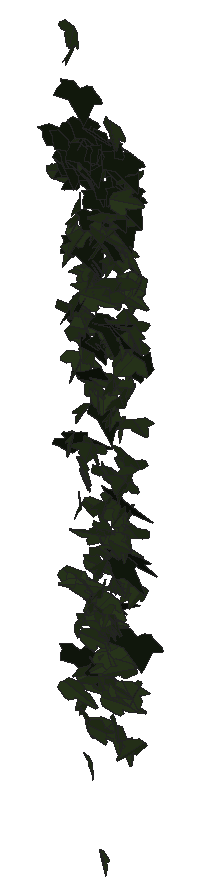
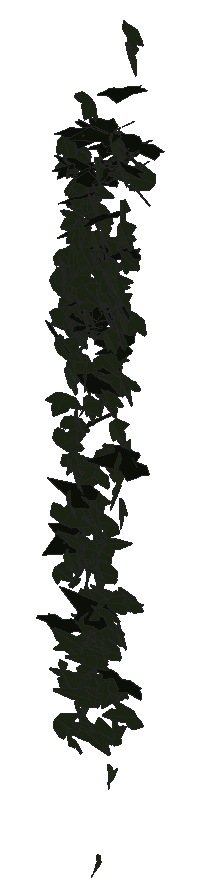
# SketchUp Ruby script. Lengths in millimetres.
U = 1.mm
M = Sketchup.active_model
def pt(a) = Geom::Point3d.new(a.map { |v| v * U })
def face(e, loops, mat)
  f = e.add_face(loops[0].map { |a| pt(a) })
  loops[1..].each { |l| e.add_face(l.map { |a| pt(a) }).erase! }
  f.material = f.back_material = mat if mat
  f
end
# faces: each face lists its corners as indices into pts; further lists are holes
def faces(e, pts, list, mat = nil) = list.each { |f| face(e, (f[0].is_a?(Array) ? f : [f]).map { |l| l.map { |i| pts[i] } }, mat) }
# xy, xz, yz: faces in a plane at the given z, y or x. An outline is a flat list of corners, or four numbers for a rectangle; further outlines are holes
def ring(l) = l.size == 4 ? [[l[0], l[1]], [l[2], l[1]], [l[2], l[3]], [l[0], l[3]]] : l.each_slice(2).to_a
def flat(e, list, mat, &to3) = list.each { |f| face(e, (f[0].is_a?(Array) ? f : [f]).map { |l| ring(l).map { |u, v| to3.(u, v) } }, mat) }
def xy(e, z, list, mat = nil) = flat(e, list, mat) { |x, y| [x, y, z] }
def xz(e, y, list, mat = nil) = flat(e, list, mat) { |x, z| [x, y, z] }
def yz(e, x, list, mat = nil) = flat(e, list, mat) { |y, z| [x, y, z] }
def lines(e, pts, list) = list.each { |a, b| e.add_line(pt(pts[a]), pt(pts[b])) }
# prism: a flat outline (further loops are holes) pulled along v
def prism(e, loops, v, mat = nil)
  f = face(e, loops, mat); d = Geom::Vector3d.new(v.map { |x| x * U })
  f.pushpull(f.normal.samedirection?(d) ? d.length : -d.length)
end
def box(e, o, s, mat = nil) = prism(e, [[o, [o[0] + s[0], o[1], o[2]], [o[0] + s[0], o[1] + s[1], o[2]], [o[0], o[1] + s[1], o[2]]]], [0, 0, s[2]], mat)
def at(x, y, z, deg = 0) = Geom::Transformation.translation(pt([x, y, z])) * Geom::Transformation.rotation(ORIGIN, Z_AXIS, deg.degrees)
def axes(o, x, y, z) = Geom::Transformation.new([*x, 0, *y, 0, *z, 0, *pt(o).to_a, 1])
def part(name) = M.definitions.add(name)
# library, detail: a bought-in or finely detailed component or shape, given as its bounding box
def library(name, o, s) = part(name).tap { |d| box(d.entities, o, s) }
def detail(e, o, s) = box(e.add_group.entities, o, s)
def put(e, d, t, mat = nil) = e.add_instance(d, t).tap { |i| i.material = mat if mat }
def group(e, t, mat = nil) = e.add_group.tap { |g| g.transformation = t; g.material = mat if mat }.entities
root = M.entities
M.materials.add("efeu1").color = [18, 25, 13]
M.materials.add("efeu2").color = [43, 57, 29]
c1 = part("ivyleaf_10")
p = [[0,12.8,-0.8],[-1.5,51.3,-10.9],[-4.9,51,-11.6],[-13.6,26.5,-7.3],[-13.2,15.9,-4.6],[-21.1,19.3,-7.2],
  [-29.5,16.3,-8.3],[-29.2,8.3,-6.2],[-19.7,-9.8,0.5],[-7.6,-13,4],[1,-12.2,5.8],[-0.4,51.1,-11.1],
  [-1.5,51.1,-10.9],[1,-12.4,5.9],[16.9,-12.4,3.5],[35.1,9.1,-5.1],[35,12.9,-6.1],[20.5,16.4,-4.9],
  [15.8,15,-3.8],[15.3,27.6,-7.1],[12.8,31.3,-7.8]]
faces(c1.entities,p,[[0,1,2,3,4,5,6,7,8,9,10],[11,12,0,13,14,15,16,17,18,19,20]],"efeu2")
c2 = part("ivyleaf_9")
p = [[39.1,54.8,31.7],[34.5,51.8,30.2],[-5.3,25.2,17.3],[-17.9,28.3,20.9],[-21.6,21.7,17],[-20.2,4.3,5.3],
  [-22.9,-0.3,2.5],[-17.1,-4,-0.6],[-2,-2.1,-1.2],[-0.7,-15.4,-10.1],[16.6,-22.3,-16.7],[21.1,-15.1,-12.5],
  [32.7,-10.7,-11],[46.1,-1.8,-6.6],[30.8,11.2,3.8]]
faces(c2.entities,p,[[0,1,2,3,4,5,6,7,8,9,10,11,12,13,14]],"efeu1")
put(root,c1,axes([1443.2,1009,891.5],[0.4432,-0.71141,0.02055],[0.0122,-0.01952,-0.74856],[1.35447,0.23296,0.00002]))
put(root,c1,axes([1420.9,977.9,1291.8],[0.03259,-0.22317,0.76558],[0.8664,0.63146,0.17389],[-1.2461,0.43321,0.14093]))
put(root,c2,axes([1421.4,989.4,1371.5],[-0.26237,-0.34361,-0.6958],[0.87628,0.53265,-0.35426],[1.18887,-0.46843,0.10756]))
put(root,c1,axes([1438.2,1034.8,194.6],[-0.19605,0.09852,0.6633],[0.4225,-0.62823,0.12779],[1.20428,0.23644,0.06315]))
put(root,c1,axes([1456.8,1015.2,448],[-0.06629,0.05289,0.64535],[-0.52427,-0.5861,0.03317],[1.11528,-0.27237,0.05395]))
put(root,c1,axes([1443.9,998.9,1135.7],[-0.06854,-0.55699,0.49682],[0.19163,-0.49647,-0.54931],[1.4075,0.04047,0.09898]))
put(root,c1,axes([1446.1,1007.6,1196.4],[0.07001,-0.74511,0.13637],[0.06701,-0.1347,-0.74549],[1.44009,0.04249,0.02806]))
put(root,c1,axes([1447.3,987,1547.4],[0.3478,-0.78477,-0.11098],[0.00279,0.11422,-0.80531],[1.50842,0.18073,0.02708]))
put(root,c2,axes([1467.9,980.6,1289.9],[-0.52167,0.59282,0.51746],[-0.42773,0.46615,-0.65309],[-1.43524,-0.3544,0.00655]))
put(root,c1,axes([1439,996.8,751.6],[0.58658,-0.50599,0.35522],[0.38482,-0.29258,-0.5922],[1.1119,0.36819,0.01756]))
put(root,c1,axes([1439.2,1019.2,902],[1.25724,0.17652,0.0558],[0.09848,0.02248,-0.68372],[-0.33829,0.66257,0.00833]))
put(root,c2,axes([1437.4,1001.9,1313.9],[-0.16929,-0.74088,0.20839],[-0.03156,-0.20788,-0.74616],[1.46443,-0.09013,0.00801]))
put(root,c1,axes([1422.4,1008.9,459.4],[0.55455,0.00595,0.60829],[1.15474,0.0458,-0.29108],[-0.0835,0.67292,0.01443]))
put(root,c2,axes([1425.5,1003,738.6],[0.25682,0.26931,-0.70933],[0.51907,0.65509,0.3006],[1.34751,-0.30367,0.0194]))
put(root,c1,axes([1442,991.5,1015.8],[-1.35528,0.1639,-0.25147],[0.45635,-0.07885,-0.7304],[-0.34365,-0.75107,0.02181]))
put(root,c1,axes([1452.2,1021,805.4],[-0.01871,-0.68823,0.14291],[-0.01415,-0.14281,-0.68828],[1.33771,-0.01114,-0.00528]))
put(root,c2,axes([1433.3,990.7,1314.8],[0.51571,-0.66444,-0.29611],[-0.05376,0.30614,-0.71279],[1.38342,0.25959,0.08268]))
put(root,c1,axes([1453.5,1005.5,982.2],[0.59287,-0.61086,-0.26841],[-0.11592,0.26895,-0.68278],[1.26457,0.31104,0.06325]))
put(root,c1,axes([1449.3,983.3,1585],[1.08412,-0.56149,-0.18704],[0.0272,0.27258,-0.77474],[1.12603,0.534,0.1988]))
put(root,c1,axes([1424,1011.9,231.1],[0.68955,0.00679,0.65215],[1.2245,0.11836,-0.35868],[-0.20312,0.73658,0.05162]))
put(root,c1,axes([1449.5,1001.3,1007.7],[0.76255,-0.54006,0.30653],[-0.24307,0.28533,0.66965],[-1.1566,-0.41603,0.06136]))
put(root,c2,axes([1434.8,990.2,1359.9],[0.2371,-0.77171,-0.14079],[0.19691,0.15748,-0.7716],[1.47991,0.10269,0.12522]))
put(root,c2,axes([1433,1013.4,969.4],[1.01094,-0.5476,0.02157],[0.02226,-0.01871,-0.76288],[1.04276,0.53129,-0.00463]))
put(root,c1,axes([1453.9,1002.9,1322.6],[0.39172,-0.74294,0.04333],[0.10233,-0.03,-0.76968],[1.41266,0.20819,0.04374]))
put(root,c2,axes([1468.2,1003.6,1319.6],[-1.41199,-0.19795,0.05758],[-0.10372,-0.01909,-0.76784],[0.3784,-0.74389,0.00438]))
put(root,c1,axes([1456,1010.5,674],[-0.48892,0.64643,0.18666],[-0.16992,0.16529,-0.69528],[-1.26923,-0.27114,0.02118]))
put(root,c2,axes([1441.8,1020,303.6],[-0.746,-0.20725,-0.62022],[1.0269,0.30604,-0.44326],[0.70316,-0.66683,-0.01067]))
put(root,c1,axes([1455.5,995.9,1234.3],[0.24112,-0.69615,-0.24596],[0.16234,0.26168,-0.69672],[1.39577,0.08983,0.12353]))
put(root,c1,axes([1460.2,1025.4,1102.2],[0.40735,-0.68514,0.11083],[0.02592,-0.11181,-0.71751],[1.32066,0.21352,-0.0201]))
put(root,c1,axes([1449.2,1004.2,369.6],[0.15642,-0.45535,-0.49981],[0.2751,-0.48002,0.46109],[-1.25707,-0.16171,0.03871]))
put(root,c1,axes([1456.4,992.5,1040.5],[0.26204,-0.65321,0.33663],[0.28255,-0.3107,-0.66361],[1.36972,0.18905,0.07249]))
put(root,c1,axes([1458.9,995.4,1166.7],[0.00847,-0.57781,0.48339],[0.20024,-0.47819,-0.57256],[1.41973,0.07089,0.07787]))
put(root,c1,axes([1463.4,1004.9,1371.8],[-0.03206,-0.77554,0.00348],[-0.00159,-0.00347,-0.77572],[1.47602,-0.01685,-0.00076]))
put(root,c2,axes([1466.8,989.6,1042.7],[-0.93135,0.42308,-0.43345],[0.63516,-0.27669,-0.64685],[-0.962,-0.59228,-0.00744]))
put(root,c1,axes([1464.8,1015.5,1090.7],[-0.5575,-0.65264,0.18639],[0.01094,-0.20539,-0.71012],[1.29172,-0.27994,0.08646]))
put(root,c1,axes([1469.6,1025.7,936.8],[-0.83095,-0.41397,0.34569],[-0.15031,-0.3909,-0.56786],[1.01538,-0.39665,0.19884]))
put(root,c1,axes([1466.1,985.2,628.7],[0.25675,-0.53892,-0.51614],[-0.03387,0.52204,-0.54972],[1.41979,0.10991,0.08022]))
put(root,c1,axes([1453,996.3,1160.3],[0.54011,0.33168,-0.70111],[0.64999,0.61686,0.43006],[1.32533,-0.4377,0.07481]))
put(root,c1,axes([1467.3,1019.1,980.4],[0.01607,-0.68794,0.11701],[-0.0117,-0.11709,-0.68796],[1.32805,0.00729,-0.00748]))
put(root,c1,axes([1462.8,1018.1,279.2],[-0.57389,-0.58911,-0.31887],[0.34056,0.26614,-0.66091],[1.22857,-0.34896,0.03425]))
put(root,c2,axes([1447.4,992.8,1331.5],[0.59078,-0.69709,-0.19095],[0.0923,0.22743,-0.75145],[1.37248,0.28476,0.13273]))
put(root,c2,axes([1450.1,986.5,1336.5],[0.43371,-0.68741,-0.30167],[0.05207,0.32266,-0.71457],[1.42777,0.19705,0.1177]))
put(root,c1,axes([1469.5,999.9,1006.1],[0.86428,-0.56948,-0.07185],[-0.07097,0.06215,-0.72831],[1.09011,0.45555,0.00954]))
put(root,c1,axes([1475.5,1008.4,737.3],[-0.99607,-0.46039,0.09507],[-0.1241,-0.06981,-0.69698],[0.88606,-0.52733,0.00926]))
put(root,c1,axes([1462.7,1013.8,1085.4],[-0.32445,0.66531,-0.22893],[0.11537,-0.22079,-0.68679],[-1.3341,-0.1809,-0.00372]))
put(root,c1,axes([1487.9,1013.6,558.6],[-0.26023,0.03474,-0.62065],[-1.07167,-0.27614,0.1086],[-0.5012,0.57241,0.09006]))
put(root,c2,axes([1461.7,992.9,1465.5],[-0.48078,-0.74161,-0.16443],[0.08133,0.15913,-0.78339],[1.44343,-0.25599,-0.01063]))
put(root,c1,axes([1458.7,1001,702.2],[-0.48312,0.46249,-0.49972],[0.4288,-0.44622,-0.52742],[-1.22288,-0.33918,0.01248]))
put(root,c1,axes([1460.7,1011.9,743.4],[-0.78915,0.50002,-0.3271],[0.4121,-0.24533,-0.64952],[-1.05988,-0.46769,-0.009]))
put(root,c1,axes([1472.6,1018.6,860.6],[1.10535,-0.27628,-0.20982],[-0.22778,0.22448,-0.62686],[0.61972,0.57528,0.14384]))
put(root,c2,axes([1486,993,1356.5],[-1.44087,0.20191,-0.12469],[0.21102,-0.06762,-0.7827],[-0.39932,-0.76429,0.03631]))
put(root,c1,axes([1471.9,1004.8,1114.1],[-0.85937,0.56141,0.074],[-0.0993,0.05299,-0.72043],[-1.07314,-0.45448,0.0074]))
put(root,c1,axes([1475.5,1020.7,1071.7],[-0.14093,-0.71007,0.10685],[-0.01513,-0.1066,-0.71392],[1.36654,-0.07441,0.00311]))
put(root,c1,axes([1443.7,1005.6,450.6],[0.39134,-0.11436,-0.72012],[1.37291,-0.07706,0.21822],[-0.20209,-0.74493,0.08798]))
put(root,c1,axes([1462.2,1007.3,180.6],[-0.59651,0.28867,0.50802],[0.71319,-0.34302,0.4261],[0.85325,0.48853,-0.001]))
put(root,c1,axes([1459.8,983,987.9],[-0.34796,-0.34077,-0.73583],[0.89725,0.56905,-0.38067],[1.25569,-0.50105,0.06811]))
put(root,c1,axes([1477.3,999.5,934.4],[0.79729,-0.48326,-0.26997],[-0.177,0.27231,-0.63176],[1.03856,0.4174,0.09958]))
put(root,c1,axes([1469.5,992,1330.6],[0.10412,0.76286,-0.02279],[-0.00187,-0.02278,-0.76482],[-1.45253,0.05471,-0.00065]))
put(root,c2,axes([1458.1,1003,1393.3],[0.49907,-0.67127,-0.29909],[-0.00908,0.316,-0.71341],[1.39861,0.24158,0.10209]))
put(root,c2,axes([1463.1,1003.5,1149.9],[-0.50102,-0.56288,-0.47031],[0.43311,0.41236,-0.62089],[1.32712,-0.34707,0.02507]))
put(root,c1,axes([1475.3,1025.1,1038.3],[0.68222,-0.60648,0.06114],[0.04696,-0.05643,-0.70446],[1.15916,0.35923,-0.00744]))
put(root,c1,axes([1482.4,1003.4,1068.7],[-0.67489,-0.56352,0.25401],[-0.11591,-0.25957,-0.66086],[1.17069,-0.35056,0.081]))
put(root,c1,axes([1476.9,1006,1117.6],[-0.9642,0.51359,0.07012],[-0.08621,0.05381,-0.72139],[-0.98276,-0.50861,-0.00551]))
put(root,c2,axes([1491.3,990.5,962.7],[0.68822,0.02148,-0.6927],[-1.31893,0.00382,-0.36165],[-0.01246,0.7814,0.02081]))
put(root,c1,axes([1483.7,1006,1106.7],[-0.57669,-0.61327,0.24037],[0.03656,-0.2727,-0.67153],[1.25309,-0.27428,0.13021]))
put(root,c1,axes([1488.3,1018.1,422.3],[1.13171,-0.21924,-0.29688],[-0.5257,0.10899,-0.63374],[0.46583,0.65563,0.00608]))
put(root,c1,axes([1481.8,1015.4,569.2],[-0.55508,0.60031,0.10335],[-0.11172,0.08635,-0.66724],[-1.15392,-0.29713,0.01489]))
put(root,c1,axes([1487.9,1014.6,1107.6],[-0.31374,-0.63964,0.30856],[-0.07828,-0.30763,-0.65969],[1.34933,-0.16657,0.03347]))
put(root,c1,axes([1485.5,1012,1184],[0.37967,-0.73235,-0.03365],[-0.01388,0.03289,-0.75903],[1.3952,0.19962,0.00161]))
put(root,c1,axes([1471.5,1011.4,87.9],[-0.37319,0.0677,0.65477],[0.77471,-0.52445,0.17612],[0.98456,0.43833,0.10961]))
put(root,c1,axes([1461.5,1024.7,608.7],[-0.39439,0.09072,-0.63142],[1.07466,-0.2828,-0.22595],[-0.56485,-0.60139,0.011]))
put(root,c1,axes([1480.3,1008.4,1095.9],[0.37984,-0.57233,0.42674],[0.30425,-0.39602,-0.6059],[1.32421,0.25516,0.0168]))
put(root,c1,axes([1464.8,1012.2,254.8],[0.75976,0.02486,-0.58698],[1.00609,0.29446,0.37199],[0.4879,-0.64591,0.14699]))
put(root,c1,axes([1492.8,1000.3,834],[0.12538,0.27428,-0.67419],[-0.13268,0.67621,0.26829],[1.37888,0.04013,0.08712]))
put(root,c1,axes([1463.5,1021.7,276.7],[-0.29689,0.01189,0.72121],[1.34588,-0.14288,0.15531],[0.27052,0.72392,0.01881]))
put(root,c2,axes([1478.4,1012.4,871],[1.40141,0.00783,0.21599],[-0.41119,0.00592,0.73634],[0.01113,-0.76735,0.00788]))
put(root,c1,axes([1485,1005.2,427.6],[-0.18719,-0.24476,-0.67812],[0.44494,0.63659,-0.26367],[1.29794,-0.25352,-0.00741]))
put(root,c1,axes([1465,1011.4,347.2],[0.14727,0.00514,0.66847],[1.23433,0.16251,-0.07633],[-0.30835,0.65301,0.01374]))
put(root,c1,axes([1475.1,1010.3,390.4],[-1.05334,-0.08744,-0.51833],[0.97325,0.08463,-0.56031],[0.23153,-0.75353,-0.00279]))
put(root,c2,axes([1481.7,990.8,1348.4],[-0.33793,-0.71373,-0.27923],[0.11589,0.27258,-0.73546],[1.45401,-0.18761,-0.00628]))
put(root,c1,axes([1493.7,1011.5,269.6],[-1.06274,-0.41819,-0.1508],[0.23417,0.08727,-0.69762],[0.81301,-0.57178,0.00381]))
put(root,c1,axes([1497.7,997.5,1158.1],[0.25738,-0.7155,-0.24789],[-0.06821,0.24548,-0.72811],[1.43954,0.13956,0.00982]))
put(root,c1,axes([1501.8,1024.1,172.5],[1.15359,-0.02355,-0.29756],[-0.56599,0.01021,-0.60659],[0.04881,0.67515,-0.0012]))
put(root,c1,axes([1491.8,1023.6,842],[0.54627,0.59829,-0.1598],[-0.11876,-0.14729,-0.66353],[-1.17257,0.29364,-0.00724]))
put(root,c1,axes([1498.5,1016.7,1166.3],[0.12014,-0.75009,-0.02448],[0.00406,0.02474,-0.75273],[1.42832,0.06302,0.0042]))
put(root,c2,axes([1481.7,1004.6,1295.5],[0.22715,-0.70852,0.26439],[0.03081,-0.26521,-0.71802],[1.43895,0.11752,-0.02636]))
put(root,c2,axes([1481.7,1005.3,1213.4],[0.23488,-0.63823,-0.40495],[0.06589,0.41465,-0.64298],[1.43704,0.0853,0.09567]))
put(root,c2,axes([1475.9,1004.7,1382],[1.38059,-0.27976,-0.0358],[0.12212,0.25992,-0.73081],[0.52271,0.67819,0.26532]))
put(root,c1,axes([1518.2,1007.2,582.3],[-0.61481,0.10404,0.5461],[-0.98137,0.17997,-0.33931],[-0.3954,-0.60844,-0.00699]))
put(root,c1,axes([1473.8,1011.4,499.3],[0.02011,-0.04651,0.69636],[1.2907,0.16514,0.00074],[-0.31366,0.67658,0.04769]))
put(root,c1,axes([1508.2,1026.6,1063.5],[-0.70213,-0.51319,0.36236],[-0.17373,-0.37197,-0.61974],[1.18296,-0.35923,0.12406]))
put(root,c1,axes([1518.1,1007.9,361.1],[0.36364,-0.15762,-0.59616],[-0.85167,0.39397,-0.24758],[0.80746,0.48652,0.00734]))
put(root,c1,axes([1494.5,1001.7,491.6],[0.29916,-0.64001,-0.20308],[0.12189,-0.19332,0.65885],[-1.27208,-0.16904,0.01537]))
put(root,c2,axes([1490.4,1027.5,805.1],[-0.02816,-0.75112,0.18296],[0.02991,-0.18325,-0.75103],[1.47102,-0.01065,0.01877]))
put(root,c1,axes([1503.9,1005.3,1306.2],[0.23302,-0.73575,-0.17778],[0.0798,0.18641,-0.74258],[1.43837,0.10885,0.07]))
put(root,c1,axes([1506.1,1007.5,635.2],[-0.21553,-0.62591,-0.07851],[0.02056,0.07783,-0.63607],[1.2004,-0.11372,-0.0032]))
put(root,c1,axes([1497.3,1013.1,-87.4],[-0.1945,0.53332,-0.33609],[0.1251,-0.32961,-0.54301],[-1.19321,-0.12149,-0.00215]))
put(root,c1,axes([1508.6,1030.5,402.6],[-0.18708,-0.54603,0.41116],[-0.06292,-0.4111,-0.55386],[1.29936,-0.09852,0.03238]))
put(root,c1,axes([1486.5,988.4,1054.3],[0.30282,0.18928,0.74365],[0.69884,0.64809,-0.24353],[-1.28238,0.39788,0.0429]))
put(root,c1,axes([1483.9,1028,376.1],[-0.15756,0.07986,0.75173],[1.22412,-0.38991,0.11226],[0.75598,0.64801,-0.0251]))
put(root,c1,axes([1514.8,1021.8,310.1],[0.43215,0.3104,-0.62414],[-0.75259,-0.48321,-0.38418],[-1.09252,0.45564,0.01776]))
put(root,c1,axes([1483,1006.2,409.1],[-0.38011,-0.04855,0.73188],[1.32196,-0.25623,0.17255],[0.44852,0.71406,0.11168]))
put(root,c1,axes([1534,1009.7,882],[-0.02132,0.05609,-0.73815],[-1.39931,0.08515,0.01763],[0.16411,0.73331,0.05442]))
put(root,c1,axes([1499.2,1015.8,694.1],[-1.08527,0.08825,-0.28166],[0.51692,-0.08298,-0.57587],[-0.21991,-0.63057,0.03637]))
put(root,c1,axes([1512.9,999.6,513.5],[0.42357,-0.29941,0.51724],[-0.50566,0.44483,0.37182],[-1.01887,-0.34524,0.0305]))
put(root,c1,axes([1515.5,1020.5,631.1],[0.89421,-0.55043,-0.28111],[-0.35372,0.21094,-0.72368],[1.12184,0.50525,-0.00411]))
put(root,c1,axes([1513.4,1008.1,443.3],[1.14149,-0.08531,-0.20905],[-0.39464,0.02668,-0.60581],[0.17005,0.6346,-0.00263]))
put(root,c2,axes([1482.3,1019.8,415.5],[1.17273,0.35231,-0.28515],[0.45287,0.15814,0.70957],[0.73419,-0.6603,0.0178]))
put(root,c1,axes([1499,1008.4,537.1],[-0.85517,-0.1857,-0.41301],[0.71657,0.17006,-0.48609],[0.47884,-0.58614,-0.01018]))
put(root,c1,axes([1483.3,1008.4,388],[0.22875,-0.0061,-0.71282],[1.35553,0.03094,0.11983],[0.05614,-0.72222,0.01115]))
put(root,c2,axes([1516.6,1002,1373.3],[-1.34912,-0.15793,-0.29073],[0.56802,-0.00854,-0.72306],[0.27178,-0.76612,0.068]))
put(root,c1,axes([1511.5,1009.9,702.3],[-0.89861,0.42684,-0.06049],[0.07845,-0.0446,-0.63647],[-0.81672,-0.47392,0.00542]))
put(root,c2,axes([1530.3,1006.1,965.4],[-1.03263,-0.55871,0.11639],[0.17401,0.07342,0.77868],[-1.07213,0.55004,0.01428]))
put(root,c1,axes([1517.9,984.6,475.9],[-0.00354,-0.64236,-0.35691],[-0.0121,0.35691,-0.64233],[1.39852,0.00146,-0.00646]))
put(root,c1,axes([1518.3,1024.2,1128.3],[-0.18922,-0.68694,0.23503],[0.01772,-0.23841,-0.69288],[1.38167,-0.09102,0.04107]))
put(root,c1,axes([1518.9,994.5,524.8],[-0.11144,-0.77801,0.02963],[-0.00537,-0.0295,-0.78021],[1.48177,-0.05862,-0.0006]))
put(root,c1,axes([1487.3,1004.6,169.7],[0.00993,-0.07878,0.72989],[1.37415,0.13257,0.00915],[-0.25272,0.71777,0.07842]))
put(root,c1,axes([1509.9,1022.6,362.9],[-0.35789,0.38277,0.56609],[0.49151,-0.50379,0.42643],[1.20412,0.31941,-0.00581]))
put(root,c1,axes([1524.7,1002.4,1134.1],[0.3882,-0.51904,-0.48633],[-0.37634,0.44461,-0.55745],[1.30035,0.28363,-0.01615]))
put(root,c1,axes([1519.1,1008.7,1065.5],[-1.04563,-0.48068,-0.18892],[0.30424,0.10402,-0.72954],[0.93469,-0.57159,0.02611]))
put(root,c1,axes([1510.8,1002.9,390.1],[0.0365,0.05739,-0.63411],[0.60377,0.54919,0.0593],[1.05065,-0.31759,-0.01205]))
put(root,c1,axes([1528.1,999.8,479.2],[0.06242,-0.04201,0.63628],[-0.61092,0.54943,0.05282],[-1.04863,-0.32259,0.0071]))
put(root,c1,axes([1523.8,1009.5,823.7],[0.14199,-0.70159,0.00059],[-0.00104,-0.00065,-0.70554],[1.33526,0.07461,-0.00061]))
put(root,c1,axes([1525,985.5,1234.6],[0.31488,-0.61795,-0.45472],[-0.05748,0.45957,-0.63552],[1.45905,0.15146,0.07309]))
put(root,c1,axes([1501.5,1009.4,320.1],[-0.30363,-0.07535,-0.64788],[1.15621,0.2256,-0.17583],[0.45183,-0.62794,0.01457]))
put(root,c1,axes([1513,1008.1,323.4],[1.05123,0.28289,0.14096],[0.22932,0.07392,-0.62049],[-0.55611,0.56524,0.0106]))
put(root,c1,axes([1527.3,1000.3,986.9],[0.10977,-0.70058,-0.01657],[-0.01091,0.01616,-0.70294],[1.33367,0.05779,-0.00439]))
put(root,c1,axes([1517.7,990.6,1010.7],[0.92019,0.62664,0.04036],[0.04596,0.03235,-0.79148],[-1.1942,0.4841,0.00064]))
put(root,c1,axes([1526.5,1003.6,889.4],[0.06075,-0.68244,-0.38392],[0.15276,0.38507,-0.67781],[1.4824,-0.01171,0.08558]))
put(root,c1,axes([1526.8,1006.1,528.1],[0.02762,-0.12903,-0.69764],[0.14345,0.69412,-0.12681],[1.34262,-0.0715,0.0279]))
put(root,c1,axes([1522.8,1012.4,827.2],[-0.00911,0.48929,-0.55508],[-0.0284,-0.55505,-0.48912],[-1.40798,0.00803,0.01346]))
put(root,c1,axes([1528.9,992.9,1225.5],[0.65928,-0.69048,0.02761],[0.00542,-0.02945,-0.77243],[1.31517,0.34625,-0.01066]))
put(root,c1,axes([1531.1,1001.9,994.7],[0.68897,-0.59674,-0.17286],[-0.0847,0.17464,-0.69609],[1.17936,0.36115,0.05099]))
put(root,c2,axes([1508.4,995.4,991.8],[1.24413,0.41711,-0.05239],[0.08219,0.02971,0.77544],[0.79585,-0.65513,0.00182]))
put(root,c1,axes([1533.6,1018.9,1161.9],[-0.59508,-0.66254,-0.06306],[0.14295,0.0341,-0.73068],[1.25855,-0.31714,0.05317]))
put(root,c2,axes([1520.8,1001,1354.6],[-0.1036,-0.73111,-0.26218],[0.08047,0.25965,-0.73282],[1.47603,-0.06547,0.02155]))
put(root,c1,axes([1533.6,999.2,428.7],[0.40806,0.45945,-0.40181],[-0.30649,-0.36821,-0.50696],[-1.12049,0.26804,-0.00766]))
put(root,c2,axes([1519.5,997.1,1291.2],[0.29175,-0.69187,-0.32191],[-0.04731,0.32364,-0.70743],[1.45155,0.14961,0.04164]))
put(root,c2,axes([1520.1,990.6,1270.7],[-0.36739,-0.58333,-0.50813],[0.42136,0.46015,-0.61236],[1.41075,-0.28935,0.05057]))
put(root,c1,axes([1534.3,994.4,1415.2],[-1.10625,0.51723,-0.15152],[-0.01491,-0.23093,-0.75826],[-1.02565,-0.55452,0.17445]))
put(root,c1,axes([1509.3,988,1198.6],[-0.45728,0.08563,-0.74359],[1.36504,-0.19703,-0.25444],[-0.40744,-0.7562,-0.01791]))
put(root,c1,axes([1556.6,989.8,1141.6],[0.61275,-0.11346,0.72174],[-1.27889,0.2636,0.34119],[-0.54579,-0.74504,0.01081]))
put(root,c1,axes([1527.6,1030.5,796.3],[0.60292,-0.43259,0.41337],[0.47852,-0.32819,-0.53613],[1.03333,0.40438,0.00709]))
put(root,c1,axes([1514.3,1010.7,262.4],[-0.08543,-0.04702,0.64051],[1.21991,-0.04341,0.04173],[0.07639,0.64061,0.04984]))
put(root,c1,axes([1510.2,1021.2,541.8],[0.14289,-0.00656,-0.7683],[1.3755,-0.26137,0.07286],[-0.49625,-0.72636,-0.01928]))
put(root,c1,axes([1530.1,1011.5,616],[1.09091,-0.198,0.21383],[0.3874,-0.06563,-0.60641],[0.39691,0.60825,0.00417]))
put(root,c1,axes([1547,985.4,1236.8],[-1.23892,-0.54586,0.01318],[-0.0188,-0.00873,-0.84954],[1.03901,-0.65104,0.00034]))
put(root,c2,axes([1536.1,997.5,1014.1],[-0.59819,-0.69548,-0.14444],[0.12316,0.12925,-0.76319],[1.34627,-0.32085,0.00564]))
put(root,c2,axes([1560.8,1012.7,1297.2],[-1.42429,-0.07417,0.10492],[-0.19575,-0.02579,-0.75187],[0.14655,-0.75524,0.01537]))
put(root,c1,axes([1541.7,990.7,402.1],[-1.05189,0.37791,0.20592],[0.31149,-0.12541,0.66946],[0.75754,0.57632,0.01065]))
put(root,c1,axes([1544.2,1014.3,674.8],[0.31969,-0.62768,0.07538],[0.05271,-0.07061,-0.64971],[1.20202,0.17004,0.00844]))
put(root,c1,axes([1552.3,998.6,980.1],[-0.50779,-0.58561,0.33355],[-0.21349,-0.31514,-0.64303],[1.26475,-0.28832,0.02538]))
put(root,c1,axes([1516.8,1011.1,235.3],[0.03847,0.03301,0.75523],[1.29319,0.33031,-0.03263],[-0.63054,0.67946,-0.02083]))
put(root,c1,axes([1549.5,1001.2,1161.9],[0.57391,-0.49517,-0.51072],[-0.1893,0.51991,-0.56281],[1.34055,0.28541,0.13917]))
put(root,c1,axes([1556.6,1000.9,695.3],[-1.11684,-0.11813,0.23916],[-0.4324,-0.08145,-0.59771],[0.26598,-0.62843,0.03251]))
put(root,c2,axes([1517.3,1021.7,640.5],[0.64824,-0.33455,0.60485],[0.79412,-0.43806,-0.47726],[1.04876,0.53848,-0.01247]))
put(root,c1,axes([1531.6,1003.2,195.5],[0.00929,-0.19008,0.68278],[0.8881,-0.51305,-0.14617],[1.01526,0.45054,0.12161]))
put(root,c1,axes([1550.6,1006.6,1169.6],[-0.51109,0.59943,0.34639],[-0.35547,0.29504,-0.65535],[-1.26876,-0.32412,0.04407]))
put(root,c1,axes([1546,1020.1,463.5],[-0.33559,0.40716,0.56258],[0.25859,-0.54899,0.43991],[1.29615,0.21494,0.05789]))
put(root,c1,axes([1547.4,1010.4,623.4],[0.09197,0.1535,-0.66955],[-0.23483,-0.65835,-0.15984],[-1.28608,0.13118,-0.01869]))
put(root,c1,axes([1551.4,1022.8,514.7],[-0.10366,-0.67467,0.07165],[-0.00511,-0.07167,-0.67685],[1.29124,-0.05445,0.00307]))
put(root,c2,axes([1532,997.2,1173.2],[0.82291,-0.58718,-0.2582],[-0.13259,0.26656,-0.72284],[1.21358,0.42729,0.09611]))
put(root,c1,axes([1555.7,998.9,1229.4],[-0.15377,-0.60541,0.47373],[-0.11372,-0.46995,-0.61078],[1.45862,-0.10046,0.00232]))
put(root,c1,axes([1562.4,1021.1,584.4],[-1.15846,-0.21908,-0.35197],[-0.60432,-0.15565,0.64601],[-0.50731,0.68568,0.03419]))
put(root,c1,axes([1547.2,1028.7,893.4],[0.45308,-0.54052,0.34973],[0.26171,-0.32157,-0.59061],[1.19698,0.2749,-0.00324]))
put(root,c1,axes([1550.6,988.9,1107.3],[-1.20495,-0.44401,-0.19405],[0.3022,0.11154,-0.77329],[0.87129,-0.65272,-0.00015]))
put(root,c2,axes([1528.9,997.3,990.2],[0.20808,-0.25705,0.78758],[0.51017,-0.7407,-0.27896],[1.49192,0.28914,-0.01445]))
put(root,c1,axes([1574.1,1010.9,984.8],[-1.01731,-0.06601,0.52385],[-0.97147,-0.12602,-0.53672],[0.25697,-0.73774,0.0448]))
put(root,c1,axes([1566.4,999.3,321.4],[-0.26697,-0.21471,0.59454],[-0.53548,-0.52415,-0.25567],[1.07731,-0.31374,0.02025]))
put(root,c1,axes([1547.3,1028.6,626.8],[0.50048,-0.52173,0.42454],[0.38034,-0.37465,-0.5842],[1.22236,0.33019,0.00795]))
put(root,c1,axes([1535.7,1025.5,698.9],[0.30414,-0.21747,0.57718],[0.94221,-0.31039,-0.25402],[0.70014,0.51218,0.09113]))
put(root,c1,axes([1542.1,999,187.4],[0.9596,-0.41362,0.3634],[0.56537,-0.21051,-0.65176],[0.88225,0.58478,0.02241]))
put(root,c1,axes([1535.9,996,492.7],[-0.15077,0.03285,0.69201],[1.0471,-0.42031,0.08294],[0.80129,0.55543,0.02183]))
put(root,c1,axes([1557,1020.2,875.2],[0.25514,-0.68369,0.04869],[0.00431,-0.04917,-0.69667],[1.30449,0.13388,-0.00722]))
put(root,c1,axes([1568.5,1019.5,919.5],[-1.07393,0.28334,-0.29229],[-0.50296,0.12503,0.63139],[0.5893,0.62306,0.00622]))
put(root,c1,axes([1555.8,1005,1106.4],[-0.06593,-0.66941,-0.28687],[0.13695,0.28264,-0.66823],[1.37929,-0.06006,0.05264]))
put(root,c2,axes([1544.1,1004.9,1227.7],[-0.09596,-0.75448,-0.14466],[0.04666,0.14332,-0.75602],[1.46133,-0.05412,0.01464]))
put(root,c1,axes([1562.8,1003.1,969.1],[-0.17727,-0.66189,0.35511],[-0.08352,-0.35242,-0.6684],[1.42712,-0.10285,0.00499]))
put(root,c1,axes([1544.9,1025.1,151.1],[0.80784,-0.31752,0.4452],[0.66294,-0.27744,-0.52998],[0.80225,0.549,-0.01035]))
put(root,c1,axes([1537.9,996.6,571],[0.10705,-0.17617,-0.67575],[0.87091,-0.50281,0.16917],[-1.00397,-0.45496,0.0747]))
put(root,c1,axes([1569.6,989,760.3],[-1.09662,0.18721,0.25815],[-0.46291,0.08676,-0.60581],[-0.39248,-0.6254,-0.00677]))
put(root,c1,axes([1545,1015.7,269.1],[1.19463,0.25171,0.32357],[0.57731,0.11286,-0.67625],[-0.52482,0.69711,-0.00735]))
put(root,c2,axes([1543.4,1006.2,545.1],[1.48202,0.11175,0.06692],[0.12452,0.0152,-0.78665],[-0.21437,0.78142,0.00573]))
put(root,c1,axes([1562.9,997.5,699.8],[-0.1395,-0.4451,-0.52544],[0.12646,0.52137,-0.45092],[1.30447,-0.09814,-0.01248]))
put(root,c1,axes([1573.6,1010.1,728.1],[-0.65082,-0.32832,-0.55329],[-0.69078,-0.4189,0.4729],[-1.01099,0.49758,0.03305]))
put(root,c1,axes([1564.7,977.3,882.3],[-0.26318,-0.67568,-0.46651],[0.13524,0.46146,-0.68942],[1.55681,-0.15431,-0.01898]))
put(root,c1,axes([1566,996.6,992.4],[0.91446,-0.5197,-0.19845],[-0.16863,0.18738,-0.70524],[1.04523,0.48491,0.05984]))
put(root,c1,axes([1544.7,1010.5,332.9],[0.8922,0.29374,-0.55906],[0.92656,0.27541,0.55294],[0.7656,-0.67562,-0.01767]))
put(root,c1,axes([1550.4,997.2,1172],[-1.02993,0.26785,-0.43791],[0.6969,-0.24453,-0.60207],[-0.68471,-0.65179,0.04592]))
put(root,c2,axes([1552.3,997.9,1355.7],[-0.17034,-0.69705,-0.33683],[0.13437,0.33031,-0.70232],[1.46726,-0.11117,0.02521]))
put(root,c1,axes([1555,1003.3,578],[0.86612,-0.45276,0.36218],[0.51789,-0.23978,-0.64166],[0.97439,0.52989,0.0191]))
put(root,c1,axes([1562.4,1005.8,889.5],[-0.16409,0.36395,0.64719],[0.34088,-0.6221,0.37371],[1.37141,0.19818,-0.01545]))
put(root,c1,axes([1571.2,1019.7,1072.1],[-0.23683,-0.71897,0.0291],[-0.00926,-0.02869,-0.72965],[1.36942,-0.12453,0.0001]))
put(root,c1,axes([1564.3,1002,991.5],[-0.04214,-0.58779,0.48181],[0.38876,-0.46888,-0.56263],[1.39326,0.11305,0.17156]))
put(root,c1,axes([1567.3,984.6,1292.5],[-0.43092,-0.64247,-0.42657],[0.32671,0.39143,-0.68067],[1.4309,-0.28286,0.02695]))
put(root,c1,axes([1563.1,1018.4,1047.8],[0.11336,-0.3801,0.62989],[0.46905,-0.58513,-0.37639],[1.31927,0.2407,0.0797]))
put(root,c2,axes([1556.4,999.9,1283.3],[-0.0523,-0.7092,-0.31424],[0.1197,0.31136,-0.70821],[1.47144,-0.05054,0.04644]))
put(root,c1,axes([1571.6,1016.3,1108.1],[-0.59143,-0.50032,0.42625],[0.14017,-0.49503,-0.52735],[1.24305,-0.18223,0.26228]))
put(root,c1,axes([1563.4,1003.4,504.6],[0.77451,-0.44425,0.29438],[0.34394,-0.23341,-0.60207],[0.95418,0.44473,-0.02193]))
put(root,c1,axes([1576.9,995.6,1024.1],[-1.23019,-0.32422,-0.1895],[-0.30725,-0.10068,0.72293],[-0.6453,0.66602,0.01704]))
put(root,c1,axes([1574.2,994.6,955],[1.46445,-0.08721,-0.22454],[-0.42534,0.02198,-0.77438],[0.17106,0.80126,-0.00319]))
put(root,c1,axes([1578.4,1012,165.6],[-0.2066,-0.51345,0.55651],[-0.20709,-0.54578,-0.52479],[1.42613,-0.15364,0.00442]))
put(root,c1,axes([1557.5,997.5,1082],[-0.80125,-0.35916,-0.51242],[0.88844,0.23102,-0.54546],[0.7931,-0.62164,0.09335]))
put(root,c2,axes([1558.4,988,541.6],[0.48451,-0.63931,-0.38369],[-0.23025,0.36465,-0.68785],[1.40025,0.28117,0.01966]))
put(root,c1,axes([1573.2,1021.9,1101],[0.41588,-0.68342,-0.14358],[0.04235,0.15718,-0.7143],[1.32841,0.20895,0.06772]))
put(root,c1,axes([1575.9,1004.6,1323.9],[-0.33873,-0.74343,-0.04971],[0.0287,0.04751,-0.76443],[1.41777,-0.17858,0.0036]))
put(root,c1,axes([1573.5,1017.2,278.9],[0.48202,-0.63964,0.08936],[0.05372,-0.08493,-0.68794],[1.22802,0.25479,-0.00498]))
put(root,c1,axes([1567.6,1002.2,1013],[-0.98209,0.38124,-0.31785],[0.36358,-0.27064,-0.63475],[-0.8719,-0.54227,0.09333]))
put(root,c1,axes([1571.9,1015.2,818.1],[-0.85033,-0.41996,-0.24115],[0.37719,0.1408,-0.6124],[0.84095,-0.4878,0.03084]))
put(root,c2,axes([1593.1,1008.4,930.2],[-0.16359,0.32364,0.72585],[-0.32319,0.70574,-0.33479],[-1.4776,-0.1902,-0.00713]))
put(root,c1,axes([1577.3,1019.8,474.7],[-0.27867,-0.48517,0.45122],[0.10856,-0.46962,-0.48644],[1.2563,-0.06703,0.14212]))
put(root,c2,axes([1569.7,1020.1,377.4],[-0.9381,-0.46271,-0.41312],[0.56673,0.28638,-0.67605],[1.03563,-0.57586,-0.00426]))
put(root,c1,axes([1566.7,970.3,1285.5],[0.15763,0.26282,0.761],[0.2413,0.75121,-0.27324],[-1.51316,0.14717,0.0357]))
